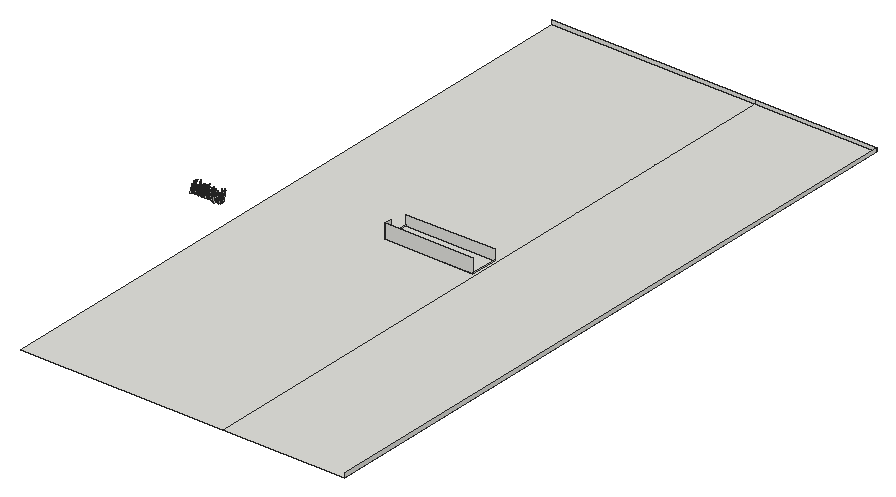
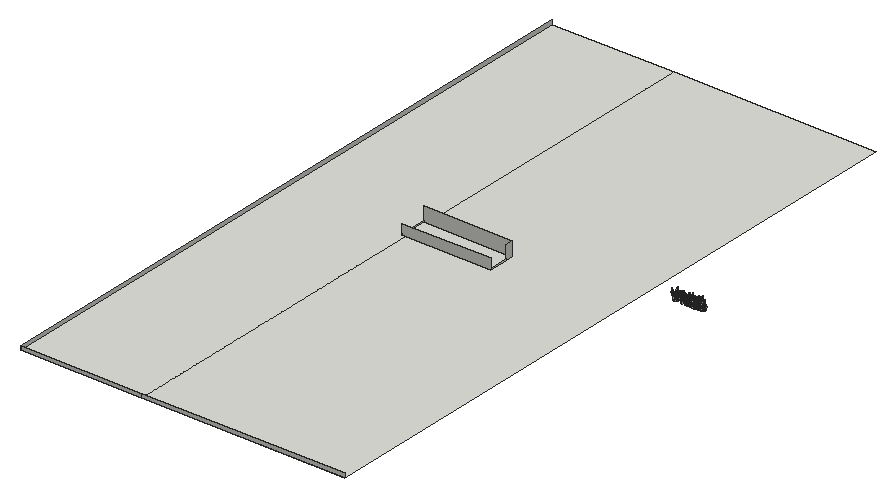
# SketchUp Ruby script. Lengths in inches.
U = 1.inch
M = Sketchup.active_model
def pt(a) = Geom::Point3d.new(a.map { |v| v * U })
def face(e, loops, mat)
  f = e.add_face(loops[0].map { |a| pt(a) })
  loops[1..].each { |l| e.add_face(l.map { |a| pt(a) }).erase! }
  f.material = f.back_material = mat if mat
  f
end
# faces: each face lists its corners as indices into pts; further lists are holes
def faces(e, pts, list, mat = nil) = list.each { |f| face(e, (f[0].is_a?(Array) ? f : [f]).map { |l| l.map { |i| pts[i] } }, mat) }
# xy, xz, yz: faces in a plane at the given z, y or x. An outline is a flat list of corners, or four numbers for a rectangle; further outlines are holes
def ring(l) = l.size == 4 ? [[l[0], l[1]], [l[2], l[1]], [l[2], l[3]], [l[0], l[3]]] : l.each_slice(2).to_a
def flat(e, list, mat, &to3) = list.each { |f| face(e, (f[0].is_a?(Array) ? f : [f]).map { |l| ring(l).map { |u, v| to3.(u, v) } }, mat) }
def xy(e, z, list, mat = nil) = flat(e, list, mat) { |x, y| [x, y, z] }
def xz(e, y, list, mat = nil) = flat(e, list, mat) { |x, z| [x, y, z] }
def yz(e, x, list, mat = nil) = flat(e, list, mat) { |y, z| [x, y, z] }
def lines(e, pts, list) = list.each { |a, b| e.add_line(pt(pts[a]), pt(pts[b])) }
# prism: a flat outline (further loops are holes) pulled along v
def prism(e, loops, v, mat = nil)
  f = face(e, loops, mat); d = Geom::Vector3d.new(v.map { |x| x * U })
  f.pushpull(f.normal.samedirection?(d) ? d.length : -d.length)
end
def box(e, o, s, mat = nil) = prism(e, [[o, [o[0] + s[0], o[1], o[2]], [o[0] + s[0], o[1] + s[1], o[2]], [o[0], o[1] + s[1], o[2]]]], [0, 0, s[2]], mat)
def at(x, y, z, deg = 0) = Geom::Transformation.translation(pt([x, y, z])) * Geom::Transformation.rotation(ORIGIN, Z_AXIS, deg.degrees)
def axes(o, x, y, z) = Geom::Transformation.new([*x, 0, *y, 0, *z, 0, *pt(o).to_a, 1])
def part(name) = M.definitions.add(name)
# library, detail: a bought-in or finely detailed component or shape, given as its bounding box
def library(name, o, s) = part(name).tap { |d| box(d.entities, o, s) }
def detail(e, o, s) = box(e.add_group.entities, o, s)
def put(e, d, t, mat = nil) = e.add_instance(d, t).tap { |i| i.material = mat if mat }
def group(e, t, mat = nil) = e.add_group.tap { |g| g.transformation = t; g.material = mat if mat }.entities
root = M.entities
c1 = part("fur_instance\#9")
p = [[0.8125,0,1.79],[0.67,-0.02,1.48],[0,-0.11,0],[0,0.11,0]]
faces(c1.entities,p,[[0,1,2,3]])
xy(root,-27.625,[[196.6875,5.77,525.63,1083.4],[525.63,5.77,722.32,1083.4]])
xy(root,-23.375,[[382.6,512.52,525.63,555.49]])
xz(root,512.52,[[382.6,-23.375,525.63,0]])
xz(root,555.49,[[382.6,-23.375,525.63,-6.4375]])
xz(root,1083.4,[[196.6875,-27.625,525.63,-21.625],[525.63,-27.625,722.32,-21.625]])
yz(root,382.6,[[512.52,-23.375,524.55,0],[524.55,-23.375,555.49,-21.625]])
yz(root,525.63,[[512.52,-23.375,555.49,-21.625]])
yz(root,722.32,[[5.77,-27.625,1083.4,-21.625]])
put(root,c1,axes([117.31,460.32,-27.1],[6.25935,-4.83068,2.00086],[-4.50057,-6.56633,-1.77386],[-2.66155,-0.25726,7.70509]))
put(root,c1,axes([127.67,458.71,-27.1],[-4.9951,-5.23204,0.99068],[-5.30492,4.77148,-1.54841],[-0.46216,1.77916,7.06595]))
put(root,c1,axes([157.9,460.79,-27.1],[-0.40558,-7.48594,0.6627],[-7.51279,0.42075,0.15485],[0.19107,0.65318,7.49532]))
put(root,c1,axes([132.0625,459.34,-27.1],[2.34766,-4.1804,1.05082],[-4.25289,-2.44131,-0.21062],[-0.70205,0.80976,4.78987]))
put(root,c1,axes([126.87,459.77,-27.1],[1.30695,-5.86281,0.96642],[-5.89292,-1.15208,0.98022],[0.76158,1.14664,5.9262]))
put(root,c1,axes([138.1875,458.29,-27.1],[2.95558,3.83246,1.3061],[4.0436,-2.87668,-0.7093],[-0.20723,-1.47175,4.78749]))
put(root,c1,axes([111.87,458.11,-27.1],[3.13745,2.7412,0.96065],[2.81213,-3.22064,0.00574],[-0.7273,-0.62763,4.16626]))
put(root,c1,axes([111.26,457.29,-27.1],[-4.2045,3.84796,1.64776],[3.68267,4.51063,-1.13666],[1.98995,-0.21727,5.58504]))
put(root,c1,axes([129.21,460.48,-27.1],[-4.78281,-0.5343,0.54387],[-0.29464,4.48183,1.81189],[0.70318,-1.75621,4.45846]))
put(root,c1,axes([148.43,457.25,-27.1],[-6.12572,-2.31991,2.2614],[-2.97153,5.95041,-1.94497],[1.2907,2.68904,6.25488]))
put(root,c1,axes([114.99,459.24,-27.1],[6.44965,-0.53992,1.19924],[-0.48241,-6.55498,-0.35669],[-1.22351,-0.26161,6.46237]))
put(root,c1,axes([150.92,456.81,-27.1],[-5.40299,1.91129,1.15946],[1.49374,5.34299,-1.84687],[1.66317,1.41036,5.42535]))
put(root,c1,axes([122.49,459.41,-27.1],[4.00541,-4.88826,1.49079],[-5.10449,-3.91872,0.86522],[-0.24835,1.7057,6.26017]))
put(root,c1,axes([113.32,460.3,-27.1],[-1.78915,-3.44674,0.35763],[-3.41457,1.82215,0.479],[0.59044,0.09337,3.85378]))
put(root,c1,axes([111.07,461.14,-27.1],[4.81338,-2.70132,0.36004],[-2.51999,-4.69011,-1.49931],[-1.0375,-1.14068,5.31205]))
put(root,c1,axes([136.88,461.37,-27.1],[-3.06964,-6.81398,0.3454],[-6.81954,3.05272,-0.38339],[-0.20825,0.47214,7.46364]))
put(root,c1,axes([157.07,458.49,-27.1],[-5.34444,-2.84039,2.21318],[-3.30562,5.4408,-0.99979],[1.42788,1.96442,5.96919]))
put(root,c1,axes([117.125,460.82,-27.1],[-5.82237,-2.50943,0.01956],[-2.48564,5.77362,0.82736],[0.34528,-0.75212,6.28591]))
put(root,c1,axes([122.29,458.7,-27.1],[3.35941,2.47012,0.56366],[2.52325,-3.34641,-0.37364],[-0.22894,-0.63632,4.15301]))
put(root,c1,axes([115.23,460.01,-27.1],[1.42662,-4.11071,0.89066],[-4.20545,-1.41051,0.22612],[-0.07357,0.91596,4.34535]))
put(root,c1,axes([144.86,457.99,-27.1],[1.84734,5.85191,0.92453],[5.8229,-1.61485,-1.41361],[1.09242,-1.28828,5.97153]))
put(root,c1,axes([153.78,459.51,-27.1],[-3.82053,1.38738,1.41647],[1.59253,3.97908,0.39802],[1.18113,-0.87734,4.0451]))
put(root,c1,axes([138.84,461.39,-27.1],[3.08843,-3.08617,0.55459],[-2.71507,-3.02147,-1.69397],[-1.56857,-0.84658,4.0241]))
put(root,c1,axes([120.125,459.5,-27.1],[-0.91503,4.79321,2.31879],[5.31141,0.98733,0.05504],[0.37492,-2.28894,4.87946]))
put(root,c1,axes([121.08,462.46,-27.1],[6.38764,-4.10189,0.26345],[-3.90919,-6.21298,-1.95294],[-1.27011,-1.50671,7.33577]))
put(root,c1,axes([140.03,459.53,-27.1],[6.60673,-3.01857,0.44503],[-3.04917,-6.49303,1.22551],[0.11127,1.29906,7.15953]))
put(root,c1,axes([113.18,458.07,-27.1],[4.04294,1.47662,0.10602],[1.40514,-3.92456,1.07725],[-0.46609,0.97696,4.16717]))
put(root,c1,axes([122.45,458.93,-27.1],[3.25743,4.86298,0.41292],[4.6269,-2.91916,-2.12138],[1.55271,-1.50328,5.4552]))
put(root,c1,axes([122.65,460.77,-27.1],[1.67883,-4.20753,0.33675],[-4.18563,-1.61266,0.71764],[0.54516,0.57551,4.47289]))
put(root,c1,axes([124.76,460.6875,-27.1],[-6.87538,0.87455,0.95023],[1.06547,6.75006,1.49673],[0.72976,-1.61573,6.76724]))
put(root,c1,axes([115.11,459.67,-27.1],[4.62251,0.92588,0.22465],[0.9419,-4.60847,-0.38752],[-0.14333,-0.42437,4.69837]))
put(root,c1,axes([114.61,459.65,-27.1],[0.94645,-5.69848,3.07489],[-6.04954,-1.88624,-1.63358],[-2.30884,2.60631,5.54074]))
put(root,c1,axes([129.4375,461.47,-27.1],[6.44633,-3.37101,0.63256],[-3.2949,-6.46051,-0.8512],[-0.95262,-0.46602,7.22457]))
put(root,c1,axes([117.5,459.28,-27.1],[3.62939,6.32437,2.66269],[6.74766,-3.83695,-0.08396],[-1.24771,-2.35377,7.2913]))
put(root,c1,axes([133.3,460.73,-27.1],[-1.38247,-3.90181,0.99129],[-3.91317,1.54858,0.63797],[0.94545,0.70412,4.09003]))
put(root,c1,axes([158.51,459.72,-27.1],[-3.07714,-3.38347,1.94932],[-3.73457,3.27489,-0.21099],[1.14047,1.59489,4.5686]))
put(root,c1,axes([125.81,463.06,-27.1],[-3.26721,-5.06008,0.08616],[-4.54982,2.98181,2.58736],[2.21606,-1.33826,5.43917]))
put(root,c1,axes([128.86,460.18,-27.1],[3.23817,-2.36152,0.30304],[-2.37388,-3.16317,0.7165],[0.18248,0.75624,3.94324]))
put(root,c1,axes([126.04,461,-27.1],[3.30583,-2.31707,0.74955],[-2.21165,-3.38553,-0.71128],[-1.01942,-0.16893,3.97384]))
put(root,c1,axes([128.5,459.23,-27.1],[2.77972,-6.83526,2.99642],[-7.05556,-1.36449,3.4327],[2.43278,3.85274,6.53179]))
put(root,c1,axes([134.58,458.43,-27.1],[1.50713,3.43781,0.3216],[3.3001,-1.53741,0.96906],[-1.01552,0.10596,3.62641]))
put(root,c1,axes([133.91,459,-27.1],[-3.45696,-5.56122,4.74392],[-6.59951,4.63089,0.61955],[3.14299,3.60698,6.51874]))
put(root,c1,axes([143.54,458.46,-27.1],[-0.09668,3.9627,0.07364],[3.92699,0.08582,0.53775],[-0.5359,-0.08606,3.92724]))
put(root,c1,axes([152.91,461.91,-27.1],[4.44508,-4.04211,0.97735],[-3.87336,-4.54492,-1.18043],[-1.51359,-0.24009,5.89101]))
put(root,c1,axes([123.89,458.59,-27.1],[3.6487,6.36792,1.23917],[6.47764,-3.65398,-0.29593],[-0.35515,-1.22351,7.3332]))
put(root,c1,axes([145.24,460.23,-27.1],[-2.81459,-5.30869,2.75415],[-5.79641,3.17103,0.18862],[1.47279,2.33491,6.00571]))
put(root,c1,axes([158.375,463.3125,-27.1],[-2.24137,-6.8028,0.2078],[-6.58087,2.22202,1.76064],[1.73594,-0.35988,6.94277]))
put(root,c1,axes([148.67,458.6,-27.1],[3.62249,2.81644,0.55831],[2.6251,-3.61284,1.19278],[-1.16313,0.61769,4.43081]))
put(root,c1,axes([125.69,459.5625,-27.1],[2.40724,3.27999,1.19788],[3.2967,-2.61439,0.53362],[-1.15108,-0.62824,4.03341]))
put(root,c1,axes([113.14,459.47,-27.1],[-4.26519,0.30143,0.24037],[0.24291,4.17451,-0.92459],[0.29939,0.9072,4.17466]))
put(root,c1,axes([143.51,459.23,-27.1],[-1.89071,3.52857,0.74513],[3.44423,2.01617,-0.80816],[1.06925,-0.25501,3.92077]))
put(root,c1,axes([119.33,460.87,-27.1],[3.22787,2.03353,0.24614],[1.96333,-2.94045,-1.45397],[0.58408,-1.35405,3.52709]))
put(root,c1,axes([146.96,461.23,-27.1],[-6.28621,2.90163,2.83322],[3.4688,6.55463,0.9835],[2.10096,-2.14018,6.85337]))
put(root,c1,axes([135.69,460.61,-27.1],[2.1664,-3.98299,1.68795],[-4.30586,-2.16689,0.41322],[-0.41582,1.68731,4.51516]))
put(root,c1,axes([150.79,460.69,-27.1],[1.73127,-4.9492,1.56465],[-4.93445,-1.0575,2.11492],[1.61056,2.08017,4.79781]))
put(root,c1,axes([124.96,460.44,-27.1],[2.68991,-2.47286,1.2383],[-2.72716,-2.65872,0.6147],[-0.45937,1.30393,3.60178]))
put(root,c1,axes([140.44,461.47,-27.1],[3.55115,-1.15094,1.45453],[-0.93925,-3.82501,-0.73353],[-1.59941,-0.30919,3.66022]))
put(root,c1,axes([130.63,461.81,-27.1],[1.50872,-3.69838,0.31644],[-3.67115,-1.43625,0.71715],[0.54852,0.55997,3.92937]))
put(root,c1,axes([156.45,463.41,-27.1],[-1.98153,-6.18192,0.39554],[-6.00617,2.01899,1.46585],[1.5161,-0.08133,6.32408]))
put(root,c1,axes([122.6,459.05,-27.1],[-0.90144,4.87523,0.09791],[4.65666,0.89022,-1.45364],[1.44671,0.1723,4.73998]))
put(root,c1,axes([148.72,459.42,-27.1],[6.05789,3.57549,2.196],[3.19122,-6.43003,1.66595],[-2.72445,0.41853,6.83424]))
put(root,c1,axes([144.8,460.93,-27.1],[5.13574,3.88277,2.0176],[4.11622,-5.34233,-0.19668],[-1.48436,-1.3806,6.4353]))
put(root,c1,axes([120.81,459.69,-27.1],[5.6278,2.51424,1.57514],[2.22036,-5.80941,1.3399],[-1.96786,0.63554,6.01649]))
put(root,c1,axes([127.95,461.3125,-27.1],[-0.77592,-4.15559,2.31409],[-4.39268,1.52537,1.26634],[1.82437,1.90534,4.03328]))
put(root,c1,axes([113.79,462.62,-27.1],[-5.15951,-5.90719,2.53837],[-5.9684,5.61072,0.92562],[2.3909,1.25844,7.78837]))
put(root,c1,axes([147.13,460.97,-27.1],[-4.91979,-5.33902,1.78444],[-5.59743,4.38767,-2.30455],[-0.5985,2.85253,6.88466]))
put(root,c1,axes([136.66,465.24,-27.1],[-6.90134,-2.30385,2.57209],[-0.73953,6.60101,3.92832],[3.37291,-3.26662,6.12409]))
put(root,c1,axes([138.62,464.64,-27.1],[-4.47086,-3.62986,0.22446],[-3.11938,4.01034,2.72058],[1.8697,-1.98902,5.07572]))
put(root,c1,axes([141.96,461.64,-27.1],[5.92157,-1.3609,0.111],[-1.36516,-5.91048,0.36315],[-0.02664,0.3788,6.06507]))
put(root,c1,axes([129.41,461.625,-27.1],[-1.9475,3.70978,1.3462],[3.85912,1.47603,1.51527],[-0.82582,-1.85103,3.9063]))
put(root,c1,axes([136.31,461.8125,-27.1],[2.61538,-3.98544,0.72253],[-3.93735,-2.29982,1.56655],[0.95028,1.43982,4.50221]))
put(root,c1,axes([146.74,459.43,-27.1],[4.8815,3.3845,2.02519],[2.72156,-5.22275,2.16824],[-2.85471,0.80828,5.53015]))
put(root,c1,axes([131.45,463.14,-27.1],[-1.6318,-4.41068,0.10105],[-4.3461,1.58854,-0.8456],[-0.75876,0.38671,4.62621]))
put(root,c1,axes([142.375,461.71,-27.1],[-2.65217,1.9255,1.58872],[2.09556,2.97695,-0.10973],[1.35655,-0.83418,3.2756]))
put(root,c1,axes([146,462.23,-27.1],[0.28341,4.29415,2.46111],[4.89058,0.13603,-0.80051],[0.76092,-2.47364,4.22839]))
put(root,c1,axes([115.875,460.25,-27.1],[-4.53452,6.13099,1.20513],[6.2123,4.58336,0.05748],[0.66981,-1.00349,7.62546]))
put(root,c1,axes([119.76,461.31,-27.1],[-4.39525,1.44739,0.73649],[1.42922,4.45652,-0.22883],[0.77116,-0.01,4.62177]))
put(root,c1,axes([151.11,464.59,-27.1],[-5.31992,-4.92486,0.01845],[-4.88394,5.27914,0.91325],[0.63384,-0.65774,7.19179]))
put(root,c1,axes([139.6875,461.125,-27.1],[3.18185,3.17768,0.5905],[3.1987,-3.21478,0.06397],[-0.46337,-0.37158,4.49642]))
put(root,c1,axes([144.24,464.07,-27.1],[2.99312,-6.69994,0.30324],[-6.59145,-2.87731,1.48788],[1.23852,0.87852,7.18569]))
put(root,c1,axes([152.43,460.02,-27.1],[-4.53148,2.02632,0.31118],[1.79338,4.28391,-1.78018],[0.99329,1.50971,4.63371]))
put(root,c1,axes([126.78,461.83,-27.1],[0.00954,3.59248,1.3323],[3.47361,-0.5704,1.51319],[-1.6171,-1.20405,3.25826]))
put(root,c1,axes([128.93,462.82,-27.1],[-2.91318,-3.12111,0.33199],[-3.12229,2.8354,-0.74159],[-0.32068,0.74655,4.20452]))
put(root,c1,axes([139.23,462.57,-27.1],[4.09073,2.15745,2.5023],[2.51133,-4.61824,-0.12369],[-2.14694,-1.2913,4.62314]))
put(root,c1,axes([127.3,461.91,-27.1],[6.46627,-2.11143,1.67342],[-2.36842,-6.52888,0.91405],[-1.28416,1.40953,6.74057]))
put(root,c1,axes([109.21,462.8125,-27.1],[3.50419,-7.42751,1.71848],[-7.22357,-2.63012,3.36199],[2.43745,2.88357,7.49295]))
put(root,c1,axes([138.99,465.61,-27.1],[-4.31312,-2.31019,0.44376],[-1.59331,3.55068,2.99849],[1.73068,-2.4885,3.8664]))
put(root,c1,axes([143.48,461.76,-27.1],[6.82569,-2.14516,0.01525],[-2.06759,-6.56497,1.95405],[0.57187,1.86856,6.88284]))
put(root,c1,axes([145.48,460.51,-27.1],[0.70112,8.01126,1.73468],[7.49163,-1.33281,3.12731],[-3.32639,-1.31314,7.4089]))
put(root,c1,axes([137.25,462.89,-27.1],[6.44978,-0.00096,0.92482],[0.04605,-6.50733,-0.32793],[-0.92367,-0.33115,6.44144]))
put(root,c1,axes([144.21,463.47,-27.1],[6.7511,0.38921,2.10678],[0.68602,-6.99103,-0.90679],[-2.02963,-1.06837,6.70124]))
put(root,c1,axes([129.51,461.69,-27.1],[4.38555,-0.36882,0.03632],[-0.36139,-4.16033,1.38975],[0.08213,1.3878,4.17584]))
put(root,c1,axes([112.98,465.71,-27.1],[-1.84089,-7.99139,1.4242],[-7.16502,2.28604,3.56596],[3.81486,0.4373,7.3848]))
put(root,c1,axes([140.45,463.99,-27.1],[-2.2334,-3.12116,0.78897],[-3.02774,2.36275,0.77617],[1.09405,0.16724,3.75863]))
put(root,c1,axes([141.28,463.07,-27.1],[-3.78552,-3.06993,0.30173],[-3.01727,3.58565,-1.37288],[-0.64154,1.25071,4.67652]))
put(root,c1,axes([158.9375,462.82,-27.1],[-3.53185,-5.19128,1.06072],[-4.89285,2.7062,-3.04713],[-2.03336,2.50511,5.48984]))
put(root,c1,axes([112.15,461.96,-27.1],[3.861,5.57007,1.34937],[5.71182,-3.87341,-0.35436],[-0.47072,-1.31331,6.76812]))
put(root,c1,axes([153.37,462.9,-27.1],[3.76786,2.01641,1.4087],[2.07515,-3.9894,0.15999],[-1.32064,-0.51569,4.27049]))
put(root,c1,axes([119.64,463.9,-27.1],[2.07826,-5.21506,0.82935],[-4.82149,-1.51054,2.58366],[2.15357,1.65083,4.98405]))
put(root,c1,axes([136.06,463.32,-27.1],[1.52671,4.77623,1.67607],[4.63081,-0.61106,-2.47682],[2.04382,-2.18327,4.35989]))
put(root,c1,axes([141.57,463.34,-27.1],[-0.36242,4.3186,2.109],[4.6668,0.82166,-0.88056],[1.14855,-1.97588,4.24338]))
put(root,c1,axes([124.36,464.97,-27.1],[-2.66612,-3.28273,0.28859],[-3.19335,2.6653,0.81637],[0.81369,-0.29607,4.14946]))
put(root,c1,axes([124.3,461.46,-27.1],[2.11808,6.39246,0.96016],[6.39192,-2.22182,0.69185],[-0.96378,-0.68681,6.6986]))
put(root,c1,axes([129.39,463.67,-27.1],[4.62058,2.87983,1.50344],[3.15499,-4.60106,-0.88304],[-0.77446,-1.56215,5.37246]))
put(root,c1,axes([145.62,462.13,-27.1],[-3.34888,5.66427,0.75226],[5.70524,3.26636,0.80369],[-0.31635,-1.05439,6.53093]))
put(root,c1,axes([117.57,464.45,-27.1],[-0.73911,-5.79285,1.55471],[-5.99778,0.70592,-0.22109],[-0.03032,1.57006,5.83563]))
put(root,c1,axes([136.09,465.99,-27.1],[-7.13222,-2.21187,1.52983],[-1.72076,7.08542,2.22194],[2.06682,-1.73369,7.12909]))
put(root,c1,axes([123.41,462.74,-27.1],[-6.49961,-2.89491,2.26898],[-3.37847,6.5202,-1.35892],[1.4542,2.20912,6.98418]))
put(root,c1,axes([110.62,463.02,-27.1],[0.08637,4.97569,1.67082],[5.15736,0.22998,-0.95146],[0.97504,-1.65717,4.88463]))
put(root,c1,axes([138.74,461.92,-27.1],[7.17048,3.0592,0.30714],[3.02615,-7.16002,0.66735],[-0.54355,0.49421,7.76718]))
put(root,c1,axes([128.4,462.48,-27.1],[-0.17119,5.69768,1.30234],[5.83131,0.07859,0.42267],[-0.39436,-1.31119,5.68456]))
put(root,c1,axes([133.4,463.62,-27.1],[-5.24229,2.67543,1.59997],[2.88849,5.34612,0.52444],[1.17239,-1.20849,5.86212]))
put(root,c1,axes([136.55,464.37,-27.1],[-1.07299,-3.39329,1.1863],[-3.30809,1.41653,1.05972],[1.4065,0.74301,3.39746]))
put(root,c1,axes([136,462.33,-27.1],[-7.59721,-1.99805,2.32928],[-2.54922,7.5713,-1.81993],[1.70857,2.41215,7.64184]))
put(root,c1,axes([134.52,462.89,-27.1],[5.06172,0.87175,1.3003],[0.68802,-5.19178,0.80241],[-1.40619,0.59773,5.07318]))
put(root,c1,axes([134.33,465.47,-27.1],[-3.22391,-4.50813,0.36238],[-4.51102,3.23719,0.13952],[0.32445,0.21334,5.54053]))
put(root,c1,axes([113.35,462.78,-27.1],[0.59003,4.76484,1.13067],[4.77949,-0.80843,0.91275],[-1.06703,-0.9864,4.71367]))
put(root,c1,axes([115.65,463.7,-27.1],[4.51759,1.55237,1.02195],[1.60919,-4.61101,-0.10928],[-0.92991,-0.4377,4.77562]))
put(root,c1,axes([114.1,464.71,-27.1],[-0.90647,-5.11686,1.80724],[-5.12934,1.40604,1.40817],[1.7715,1.45288,5.00209]))
put(root,c1,axes([110.01,464.22,-27.1],[2.80159,-3.67069,0.58517],[-3.61323,-2.51742,1.50747],[0.87232,1.36159,4.36468]))
put(root,c1,axes([150.53,464.21,-27.1],[-2.5167,4.57974,3.46384],[4.9953,3.61127,-1.14527],[2.83182,-2.30014,5.09864]))
put(root,c1,axes([158,464.68,-27.1],[2.12208,6.92928,3.4126],[7.54208,-1.09525,-2.46604],[1.66665,-3.86645,6.81445]))
put(root,c1,axes([110.16,464.58,-27.1],[5.07227,1.20948,1.05659],[1.39553,-5.05165,-0.91676],[-0.7948,-1.15114,5.13326]))
put(root,c1,axes([144.57,464.61,-27.1],[4.26627,1.55205,0.05399],[1.49304,-4.05567,-1.39111],[0.42732,-1.32496,4.32143]))
put(root,c1,axes([143.57,462.69,-27.1],[-0.37252,4.33667,0.3989],[4.3129,0.31185,0.63743],[-0.60398,-0.44793,4.30572]))
put(root,c1,axes([126.54,465.33,-27.1],[1.54796,-4.76639,0.70367],[-4.81569,-1.50748,0.38266],[0.1508,0.78667,4.99682]))
put(root,c1,axes([116.57,464.39,-27.1],[-1.858,-4.3991,1.45242],[-4.62148,1.65138,-0.9103],[-0.32175,1.68364,4.68782]))
put(root,c1,axes([153.48,465.26,-27.1],[5.8756,3.65861,0.2575],[3.32747,-5.11292,-3.2803],[1.54262,-2.90637,6.0949]))
put(root,c1,axes([119.65,461.62,-27.1],[4.83042,2.64277,1.00625],[2.0268,-4.62442,2.4159],[-1.97202,1.72053,4.9478]))
put(root,c1,axes([123.18,464.73,-27.1],[5.25974,-3.61511,1.15521],[-3.73911,-5.27428,0.51907],[-0.65007,1.0869,6.36116]))
put(root,c1,axes([151.75,464.33,-27.1],[-6.14594,-1.15799,1.95321],[-1.28361,6.42082,-0.2323],[1.87305,0.60056,6.24977]))
put(root,c1,axes([126.36,466.12,-27.1],[4.17782,-5.39394,0.17375],[-5.37681,-4.14138,0.71959],[0.46328,0.57738,6.78461]))
put(root,c1,axes([122.23,464.45,-27.1],[-2.98009,3.50221,2.17702],[3.82104,3.35523,-0.16707],[1.55067,-1.53712,4.59549]))
put(root,c1,axes([134.39,464.32,-27.1],[4.53301,0.32886,1.81446],[0.26511,-4.88148,0.22244],[-1.82486,0.10775,4.53948]))
put(root,c1,axes([114.94,461.9,-27.1],[-7.79963,1.89477,1.60693],[1.33324,7.65978,-2.56065],[2.09639,2.17814,7.60707]))
put(root,c1,axes([127.8,463.08,-27.1],[5.12063,-0.00436,1.95562],[-0.62511,-5.19742,1.62522],[-1.85303,1.74129,4.85588]))
put(root,c1,axes([145.89,463.42,-27.1],[-3.99948,7.12267,1.32626],[7.23474,3.8453,1.16596],[-0.38726,-1.72292,8.0851]))
put(root,c1,axes([144.88,465.25,-27.1],[-3.87014,-4.65436,0.40491],[-4.4497,3.51193,-2.16136],[-1.42379,1.67578,5.65416]))
put(root,c1,axes([155.11,462.04,-27.1],[-2.23637,5.81255,0.47787],[5.16217,2.21098,-2.73477],[2.71405,0.58421,5.59536]))
put(root,c1,axes([110.86,464.1875,-27.1],[4.61104,6.12434,1.67223],[6.3457,-4.50796,-0.9879],[-0.18966,-1.93296,7.60219]))
put(root,c1,axes([125.81,465.46,-27.1],[2.0151,-5.02328,1.60572],[-5.27188,-1.87389,0.75376],[0.13771,1.76848,5.35965]))
put(root,c1,axes([122.28,465.39,-27.1],[-5.21279,-1.15752,0.50027],[-1.17064,5.23306,-0.0898],[0.46875,0.19648,5.33901]))
put(root,c1,axes([120.24,466.65,-27.1],[1.37866,-6.43403,1.32521],[-6.55871,-1.42426,-0.09169],[-0.36909,1.27608,6.57944]))
put(root,c1,axes([123.24,466.74,-27.1],[1.49707,-8.01218,1.60299],[-8.01526,-1.12338,1.87068],[1.58751,1.88383,7.93327]))
put(root,c1,axes([138.96,463.71,-27.1],[3.99187,0.97882,1.10255],[0.50795,-3.90054,1.62373],[-1.38409,1.39155,3.77579]))
put(root,c1,axes([109.92,461.51,-27.1],[7.75154,3.11882,0.30174],[2.75499,-7.16733,3.30818],[-1.4927,2.96765,7.67264]))
put(root,c1,axes([115.31,465.27,-27.1],[-7.20158,-1.52489,0.67202],[-1.60184,7.15641,-0.92717],[0.45935,1.04894,7.30263]))
put(root,c1,axes([117.04,466.78,-27.1],[-3.29784,-3.61715,1.25797],[-3.53735,3.51322,0.8285],[1.46745,0.33986,4.82422]))
put(root,c1,axes([119.68,463,-27.1],[-3.94963,4.34285,0.40783],[4.0226,3.83915,-1.92507],[1.68683,1.01332,5.54563]))
put(root,c1,axes([155.06,463.95,-27.1],[0.14678,4.73777,0.12743],[4.7339,-0.15274,0.22615],[-0.23006,-0.12022,4.73465]))
put(root,c1,axes([124.15,466.65,-27.1],[-4.11377,-6.51171,1.45116],[-6.65439,3.88319,-1.43913],[-0.47668,1.98739,7.56666]))
put(root,c1,axes([142.11,462.85,-27.1],[6.07778,0.82962,2.17123],[-0.33597,-5.70106,3.1188],[-2.29992,3.02515,5.28212]))
put(root,c1,axes([151.05,465.46,-27.1],[-1.02276,3.4571,1.0392],[3.60758,1.01767,0.16502],[0.12981,-1.04418,3.60144]))
put(root,c1,axes([154.23,466.41,-27.1],[-4.22462,-4.77942,0.40733],[-4.62488,3.91455,-2.0354],[-1.27248,1.63999,6.04544]))
put(root,c1,axes([154.84,465.63,-27.1],[-3.59286,-3.26733,2.03566],[-3.70516,3.69058,-0.61592],[1.04455,1.85261,4.81713]))
put(root,c1,axes([118.02,464.09,-27.1],[6.46332,2.41268,1.62775],[2.03661,-6.58136,1.66821],[-2.07914,1.05343,6.69422]))
put(root,c1,axes([128.95,464.91,-27.1],[4.76999,5.26227,1.90717],[5.37132,-5.00824,0.38463],[-1.57405,-1.14351,7.09199]))
put(root,c1,axes([126.68,464.62,-27.1],[2.68207,4.86571,0.6841],[4.89534,-2.71316,0.10499],[-0.42283,-0.54794,5.55496]))
put(root,c1,axes([119.82,466.09,-27.1],[-1.05184,5.80364,2.59591],[6.34975,1.09094,0.13387],[0.3189,-2.57972,5.89666]))
put(root,c1,axes([123.64,464.48,-27.1],[5.3948,4.35682,0.5893],[4.31887,-5.42625,0.57994],[-0.82254,0.08385,6.9101]))
put(root,c1,axes([153.35,466.75,-27.1],[6.11915,-4.70581,1.11272],[-4.83462,-5.98952,1.25659],[-0.09634,1.67568,7.61641]))
put(root,c1,axes([155.83,463.13,-27.1],[-4.8564,4.18897,0.42907],[3.70643,4.56321,-2.59917],[1.99849,1.71635,5.86314]))
put(root,c1,axes([128.99,466.47,-27.1],[3.01328,1.01562,1.71575],[1.06477,-3.44849,0.1713],[-1.68569,-0.36275,3.17522]))
put(root,c1,axes([130.14,466.59,-27.1],[4.42305,4.26534,0.99754],[4.37397,-4.22348,-1.33498],[0.23791,-1.64944,5.99786]))
put(root,c1,axes([142.13,466.26,-27.1],[-1.06035,5.5551,1.84187],[5.77115,1.30347,-0.60889],[0.97234,-1.67863,5.62252]))
put(root,c1,axes([144.53,465.68,-27.1],[-2.34195,3.99616,0.3444],[3.99913,2.35703,-0.15486],[0.30802,-0.21845,4.62925]))
put(root,c1,axes([152.52,465.12,-27.1],[8.0865,0.10169,1.15451],[-0.2162,-7.86244,2.20681],[-1.13864,2.21504,7.78021]))
put(root,c1,axes([134.27,465.7,-27.1],[-2.5947,5.83184,0.30944],[5.66182,2.42897,1.69778],[-1.43174,-0.96349,6.15308]))
put(root,c1,axes([115.67,466.84,-27.1],[-2.80157,3.07223,0.58027],[3.12461,2.72376,0.66487],[-0.11008,-0.87559,4.10431]))
put(root,c1,axes([134.52,466.29,-27.1],[4.0884,0.15219,0.34801],[0.0557,-3.96154,1.07814],[-0.37573,1.0688,3.94662]))
put(root,c1,axes([155.5625,466.6,-27.1],[-6.9298,2.98954,1.57704],[3.02348,7.09089,-0.15622],[1.51094,-0.47802,7.54553]))
put(root,c1,axes([156.87,466.22,-27.1],[-2.11834,3.44874,0.2067],[3.45458,2.11778,0.0692],[0.04913,-0.21236,4.04678]))
put(root,c1,axes([128.25,466.05,-27.1],[1.6055,7.88479,1.47704],[7.72527,-1.11383,-2.45126],[2.16141,-1.87581,7.66412]))
put(root,c1,axes([138.67,466.15,-27.1],[4.2696,-0.12633,0.87704],[-0.45536,-4.01534,1.6384],[-0.76014,1.6958,3.94476]))
put(root,c1,axes([154.38,465.27,-27.1],[7.47336,0.82298,1.26079],[0.38429,-7.21504,2.43175],[-1.45575,2.3203,7.11442]))
put(root,c1,axes([114.3,465.85,-27.1],[2.50136,7.65725,0.1478],[7.63522,-2.48107,-0.67805],[0.59891,-0.35058,8.02686]))
put(root,c1,axes([155.12,466.16,-27.1],[-6.41092,4.00729,0.82453],[3.32918,6.00061,-3.27831],[2.37798,2.40258,6.81256]))
